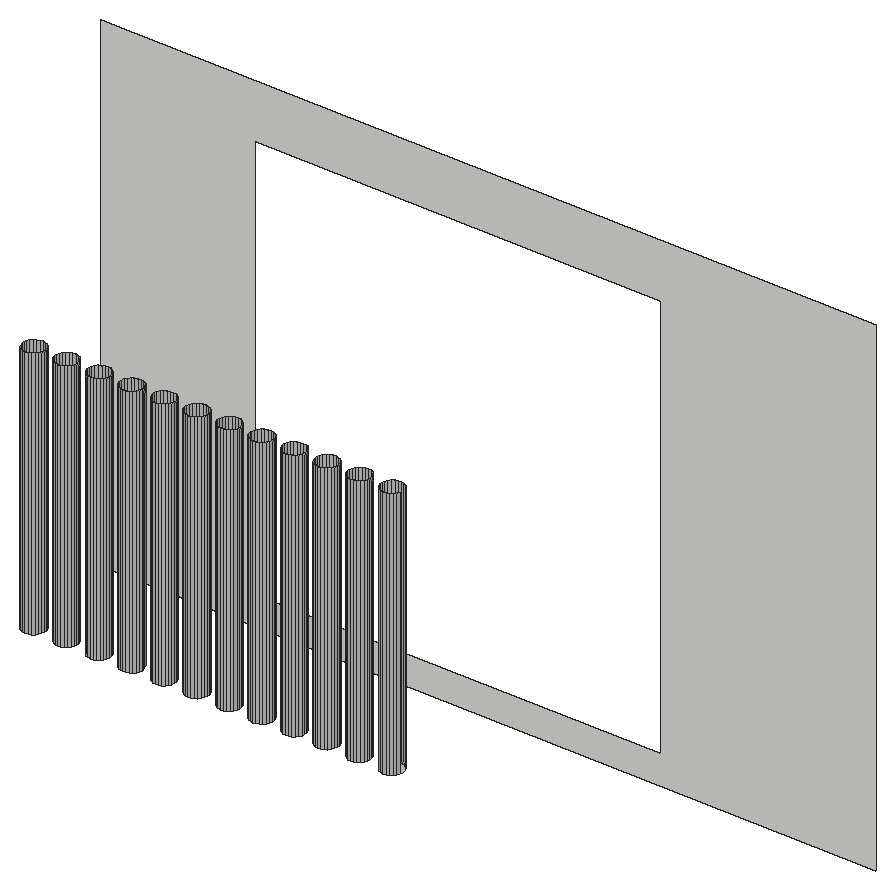
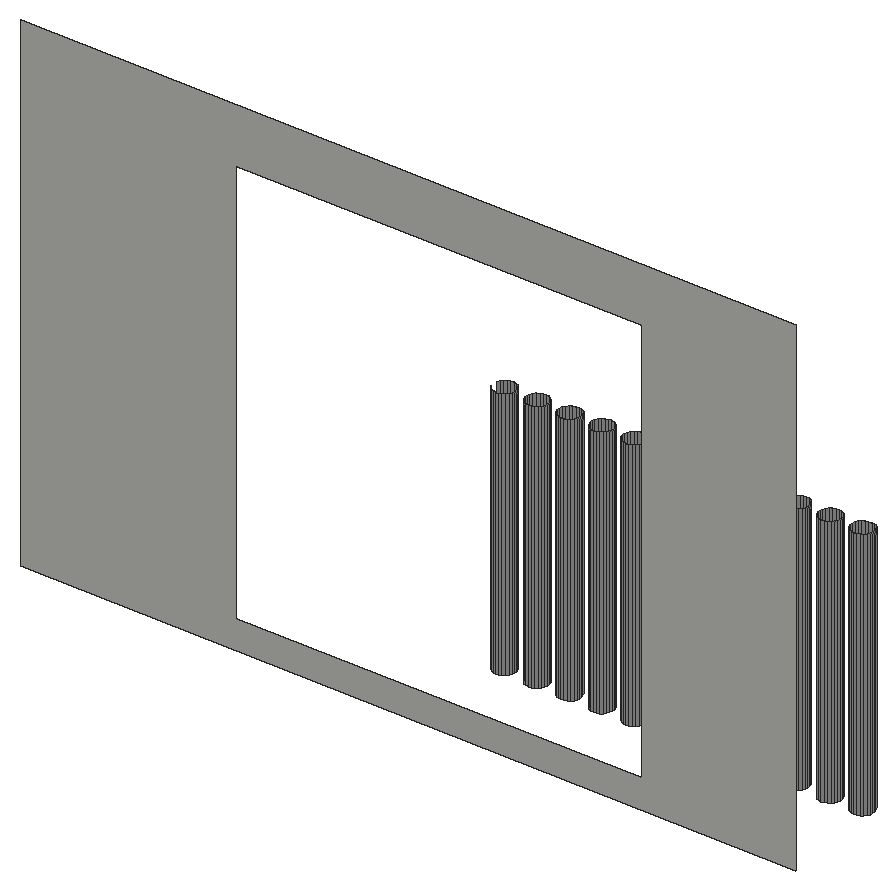
# SketchUp Ruby script. Lengths in millimetres.
U = 1.mm
M = Sketchup.active_model
def pt(a) = Geom::Point3d.new(a.map { |v| v * U })
def face(e, loops, mat)
  f = e.add_face(loops[0].map { |a| pt(a) })
  loops[1..].each { |l| e.add_face(l.map { |a| pt(a) }).erase! }
  f.material = f.back_material = mat if mat
  f
end
# faces: each face lists its corners as indices into pts; further lists are holes
def faces(e, pts, list, mat = nil) = list.each { |f| face(e, (f[0].is_a?(Array) ? f : [f]).map { |l| l.map { |i| pts[i] } }, mat) }
# xy, xz, yz: faces in a plane at the given z, y or x. An outline is a flat list of corners, or four numbers for a rectangle; further outlines are holes
def ring(l) = l.size == 4 ? [[l[0], l[1]], [l[2], l[1]], [l[2], l[3]], [l[0], l[3]]] : l.each_slice(2).to_a
def flat(e, list, mat, &to3) = list.each { |f| face(e, (f[0].is_a?(Array) ? f : [f]).map { |l| ring(l).map { |u, v| to3.(u, v) } }, mat) }
def xy(e, z, list, mat = nil) = flat(e, list, mat) { |x, y| [x, y, z] }
def xz(e, y, list, mat = nil) = flat(e, list, mat) { |x, z| [x, y, z] }
def yz(e, x, list, mat = nil) = flat(e, list, mat) { |y, z| [x, y, z] }
def lines(e, pts, list) = list.each { |a, b| e.add_line(pt(pts[a]), pt(pts[b])) }
# prism: a flat outline (further loops are holes) pulled along v
def prism(e, loops, v, mat = nil)
  f = face(e, loops, mat); d = Geom::Vector3d.new(v.map { |x| x * U })
  f.pushpull(f.normal.samedirection?(d) ? d.length : -d.length)
end
def box(e, o, s, mat = nil) = prism(e, [[o, [o[0] + s[0], o[1], o[2]], [o[0] + s[0], o[1] + s[1], o[2]], [o[0], o[1] + s[1], o[2]]]], [0, 0, s[2]], mat)
def at(x, y, z, deg = 0) = Geom::Transformation.translation(pt([x, y, z])) * Geom::Transformation.rotation(ORIGIN, Z_AXIS, deg.degrees)
def axes(o, x, y, z) = Geom::Transformation.new([*x, 0, *y, 0, *z, 0, *pt(o).to_a, 1])
def part(name) = M.definitions.add(name)
# library, detail: a bought-in or finely detailed component or shape, given as its bounding box
def library(name, o, s) = part(name).tap { |d| box(d.entities, o, s) }
def detail(e, o, s) = box(e.add_group.entities, o, s)
def put(e, d, t, mat = nil) = e.add_instance(d, t).tap { |i| i.material = mat if mat }
def group(e, t, mat = nil) = e.add_group.tap { |g| g.transformation = t; g.material = mat if mat }.entities
root = M.entities
M.materials.add("[Metal Corrugated Shiny]").color = [193, 193, 193]
xy(root,3899.4,[[7323,932.9,7306.2,935.4,7290.6,942.1,7277.2,952.6,7267.1,966.2,7260.8,982,7258.8,998.9,7261.3,1015.7,7268,1031.3,7278.5,1044.7,7292.1,1054.8,7307.9,1061.1,7324.8,1063.1,7341.6,1060.6,7357.2,1053.9,7370.6,1043.4,7380.7,1029.8,7387,1014,7389,997.1,7386.5,980.3,7379.8,964.7,7369.3,951.3,7355.7,941.2,7339.9,934.9],[7519.8,932.9,7503,935.4,7487.4,942.1,7474.1,952.6,7463.9,966.2,7457.6,982,7455.7,998.9,7458.1,1015.7,7464.8,1031.3,7475.4,1044.7,7489,1054.8,7504.8,1061.1,7521.6,1063.1,7538.5,1060.6,7554.1,1053.9,7567.4,1043.4,7577.6,1029.8,7583.8,1014,7585.8,997.1,7583.4,980.3,7576.7,964.7,7566.1,951.3,7552.5,941.2,7536.7,934.9],[7716.7,932.9,7699.9,935.4,7684.3,942.1,7670.9,952.6,7660.8,966.2,7654.5,982,7652.5,998.9,7655,1015.7,7661.7,1031.3,7672.2,1044.7,7685.8,1054.8,7701.6,1061.1,7718.5,1063.1,7735.3,1060.6,7750.9,1053.9,7764.3,1043.4,7774.4,1029.8,7780.7,1014,7782.7,997.1,7780.2,980.3,7773.5,964.7,7763,951.3,7749.4,941.2,7733.6,934.9],[7913.5,932.9,7896.7,935.4,7881.1,942.1,7867.8,952.6,7857.6,966.2,7851.3,982,7849.4,998.9,7851.8,1015.7,7858.5,1031.3,7869.1,1044.7,7882.7,1054.8,7898.5,1061.1,7915.3,1063.1,7932.2,1060.6,7947.8,1053.9,7961.1,1043.4,7971.3,1029.8,7977.5,1014,7979.5,997.1,7977.1,980.3,7970.4,964.7,7959.8,951.3,7946.2,941.2,7930.4,934.9],[8110.4,932.9,8093.6,935.4,8078,942.1,8064.6,952.6,8054.5,966.2,8048.2,982,8046.2,998.9,8048.7,1015.7,8055.4,1031.3,8065.9,1044.7,8079.5,1054.8,8095.3,1061.1,8112.2,1063.1,8129,1060.6,8144.6,1053.9,8158,1043.4,8168.1,1029.8,8174.4,1014,8176.4,997.1,8173.9,980.3,8167.2,964.7,8156.7,951.3,8143.1,941.2,8127.3,934.9],
  [8307.2,932.9,8290.4,935.4,8274.8,942.1,8261.5,952.6,8251.3,966.2,8245,982,8243.1,998.9,8245.5,1015.7,8252.2,1031.3,8262.8,1044.7,8276.4,1054.8,8292.2,1061.1,8309,1063.1,8325.9,1060.6,8341.5,1053.9,8354.8,1043.4,8365,1029.8,8371.2,1014,8373.2,997.1,8370.8,980.3,8364.1,964.7,8353.5,951.3,8339.9,941.2,8324.1,934.9],[8504.1,932.9,8487.3,935.4,8471.7,942.1,8458.3,952.6,8448.2,966.2,8441.9,982,8439.9,998.9,8442.4,1015.7,8449.1,1031.3,8459.6,1044.7,8473.2,1054.8,8489,1061.1,8505.9,1063.1,8522.7,1060.6,8538.3,1053.9,8551.7,1043.4,8561.8,1029.8,8568.1,1014,8570.1,997.1,8567.6,980.3,8560.9,964.7,8550.4,951.3,8536.8,941.2,8521,934.9],[8700.9,932.9,8684.1,935.4,8668.5,942.1,8655.2,952.6,8645,966.2,8638.7,982,8636.8,998.9,8639.2,1015.7,8645.9,1031.3,8656.5,1044.7,8670.1,1054.8,8685.9,1061.1,8702.7,1063.1,8719.6,1060.6,8735.2,1053.9,8748.5,1043.4,8758.7,1029.8,8764.9,1014,8766.9,997.1,8764.5,980.3,8757.8,964.7,8747.2,951.3,8733.6,941.2,8717.8,934.9],[8897.8,932.9,8881,935.4,8865.4,942.1,8852,952.6,8841.9,966.2,8835.6,982,8833.6,998.9,8836.1,1015.7,8842.8,1031.3,8853.3,1044.7,8866.9,1054.8,8882.7,1061.1,8899.6,1063.1,8916.4,1060.6,8932,1053.9,8945.4,1043.4,8955.5,1029.8,8961.8,1014,8963.8,997.1,8961.3,980.3,8954.6,964.7,8944.1,951.3,8930.5,941.2,8914.7,934.9],[9094.6,932.9,9077.8,935.4,9062.2,942.1,9048.9,952.6,9038.7,966.2,9032.4,982,9030.5,998.9,9032.9,1015.7,9039.6,1031.3,9050.2,1044.7,9063.8,1054.8,9079.6,1061.1,9096.4,1063.1,9113.3,1060.6,9128.9,1053.9,9142.2,1043.4,9152.4,1029.8,9158.6,1014,9160.6,997.1,9158.2,980.3,9151.5,964.7,9140.9,951.3,9127.3,941.2,9111.5,934.9],
  [9291.5,932.9,9274.7,935.4,9259.1,942.1,9245.7,952.6,9235.6,966.2,9229.3,982,9227.3,998.9,9229.8,1015.7,9236.5,1031.3,9247,1044.7,9260.6,1054.8,9276.4,1061.1,9293.3,1063.1,9310.1,1060.6,9325.7,1053.9,9339.1,1043.4,9349.2,1029.8,9355.5,1014,9357.5,997.1,9355,980.3,9348.3,964.7,9337.8,951.3,9324.2,941.2,9308.4,934.9],[9488.3,932.9,9471.5,935.4,9455.9,942.1,9442.6,952.6,9432.4,966.2,9426.1,982,9424.2,998.9,9426.6,1015.7,9433.3,1031.3,9443.9,1044.7,9457.5,1054.8,9473.3,1061.1,9490.1,1063.1,9507,1060.6,9522.6,1053.9,9535.9,1043.4,9546.1,1029.8,9552.3,1014,9554.3,997.1,9551.9,980.3,9545.2,964.7,9534.6,951.3,9521,941.2,9505.2,934.9]],"[Metal Corrugated Shiny]")
xz(root,1657.4,[[[7199.4,3899.4,11890.5,6858],[8130.9,4073.5,10586.8,6529.3]]])
p = [[7306.2,935.4,3899.4],[7323,932.9,3899.4],[7323,932.9,5423.4],[7306.2,935.4,5423.4],[7339.9,934.9,3899.4],[7339.9,934.9,5423.4],
  [7503,935.4,3899.4],[7519.8,932.9,3899.4],[7519.8,932.9,5423.4],[7503,935.4,5423.4],[7536.7,934.9,3899.4],[7536.7,934.9,5423.4],
  [7699.9,935.4,3899.4],[7716.7,932.9,3899.4],[7716.7,932.9,5423.4],[7699.9,935.4,5423.4],[7733.6,934.9,3899.4],[7733.6,934.9,5423.4],
  [7896.7,935.4,3899.4],[7913.5,932.9,3899.4],[7913.5,932.9,5423.4],[7896.7,935.4,5423.4],[7930.4,934.9,3899.4],[7930.4,934.9,5423.4],
  [8093.6,935.4,3899.4],[8110.4,932.9,3899.4],[8110.4,932.9,5423.4],[8093.6,935.4,5423.4],[8127.3,934.9,3899.4],[8127.3,934.9,5423.4],
  [8290.4,935.4,3899.4],[8307.2,932.9,3899.4],[8307.2,932.9,5423.4],[8290.4,935.4,5423.4],[8324.1,934.9,3899.4],[8324.1,934.9,5423.4],
  [8487.3,935.4,3899.4],[8504.1,932.9,3899.4],[8504.1,932.9,5423.4],[8487.3,935.4,5423.4],[8521,934.9,3899.4],[8521,934.9,5423.4],
  [8684.1,935.4,3899.4],[8700.9,932.9,3899.4],[8700.9,932.9,5423.4],[8684.1,935.4,5423.4],[8717.8,934.9,3899.4],[8717.8,934.9,5423.4],
  [8881,935.4,3899.4],[8897.8,932.9,3899.4],[8897.8,932.9,5423.4],[8881,935.4,5423.4],[8914.7,934.9,3899.4],[8914.7,934.9,5423.4],
  [9077.8,935.4,3899.4],[9094.6,932.9,3899.4],[9094.6,932.9,5423.4],[9077.8,935.4,5423.4],[9111.5,934.9,3899.4],[9111.5,934.9,5423.4],
  [9274.7,935.4,3899.4],[9291.5,932.9,3899.4],[9291.5,932.9,5423.4],[9274.7,935.4,5423.4],[9308.4,934.9,3899.4],[9308.4,934.9,5423.4],
  [9471.5,935.4,3899.4],[9488.3,932.9,3899.4],[9488.3,932.9,5423.4],[9471.5,935.4,5423.4],[9505.2,934.9,3899.4],[9505.2,934.9,5423.4],
  [7355.7,941.2,3899.4],[7355.7,941.2,5423.4],[7552.5,941.2,3899.4],[7552.5,941.2,5423.4],[7749.4,941.2,3899.4],[7749.4,941.2,5423.4],
  [7946.2,941.2,3899.4],[7946.2,941.2,5423.4],[8143.1,941.2,3899.4],[8143.1,941.2,5423.4],[8339.9,941.2,3899.4],[8339.9,941.2,5423.4],
  [8536.8,941.2,3899.4],[8536.8,941.2,5423.4],[8733.6,941.2,3899.4],[8733.6,941.2,5423.4],[8930.5,941.2,3899.4],[8930.5,941.2,5423.4],
  [9127.3,941.2,3899.4],[9127.3,941.2,5423.4],[9324.2,941.2,3899.4],[9324.2,941.2,5423.4],[9521,941.2,3899.4],[9521,941.2,5423.4],
  [7290.6,942.1,3899.4],[7290.6,942.1,5423.4],[7487.4,942.1,3899.4],[7487.4,942.1,5423.4],[7684.3,942.1,3899.4],[7684.3,942.1,5423.4],
  [7881.1,942.1,3899.4],[7881.1,942.1,5423.4],[8078,942.1,3899.4],[8078,942.1,5423.4],[8274.8,942.1,3899.4],[8274.8,942.1,5423.4],
  [8471.7,942.1,3899.4],[8471.7,942.1,5423.4],[8668.5,942.1,3899.4],[8668.5,942.1,5423.4],[8865.4,942.1,3899.4],[8865.4,942.1,5423.4],
  [9062.2,942.1,3899.4],[9062.2,942.1,5423.4],[9259.1,942.1,3899.4],[9259.1,942.1,5423.4],[9455.9,942.1,3899.4],[9455.9,942.1,5423.4],
  [7369.3,951.3,3899.4],[7369.3,951.3,5423.4],[7566.1,951.3,3899.4],[7566.1,951.3,5423.4],[7763,951.3,3899.4],[7763,951.3,5423.4],
  [7959.8,951.3,3899.4],[7959.8,951.3,5423.4],[8156.7,951.3,3899.4],[8156.7,951.3,5423.4],[8353.5,951.3,3899.4],[8353.5,951.3,5423.4],
  [8550.4,951.3,3899.4],[8550.4,951.3,5423.4],[8747.2,951.3,3899.4],[8747.2,951.3,5423.4],[8944.1,951.3,3899.4],[8944.1,951.3,5423.4],
  [9140.9,951.3,3899.4],[9140.9,951.3,5423.4],[9337.8,951.3,3899.4],[9337.8,951.3,5423.4],[9534.6,951.3,3899.4],[9534.6,951.3,5423.4],
  [7277.2,952.6,3899.4],[7277.2,952.6,5423.4],[7474.1,952.6,3899.4],[7474.1,952.6,5423.4],[7670.9,952.6,3899.4],[7670.9,952.6,5423.4],
  [7867.8,952.6,3899.4],[7867.8,952.6,5423.4],[8064.6,952.6,3899.4],[8064.6,952.6,5423.4],[8261.5,952.6,3899.4],[8261.5,952.6,5423.4],
  [8458.3,952.6,3899.4],[8458.3,952.6,5423.4],[8655.2,952.6,3899.4],[8655.2,952.6,5423.4],[8852,952.6,3899.4],[8852,952.6,5423.4],
  [9048.9,952.6,3899.4],[9048.9,952.6,5423.4],[9245.7,952.6,3899.4],[9245.7,952.6,5423.4],[9442.6,952.6,3899.4],[9442.6,952.6,5423.4],
  [7379.8,964.7,3899.4],[7379.8,964.7,5423.4],[7576.7,964.7,3899.4],[7576.7,964.7,5423.4],[7773.5,964.7,3899.4],[7773.5,964.7,5423.4],
  [7970.4,964.7,3899.4],[7970.4,964.7,5423.4],[8167.2,964.7,3899.4],[8167.2,964.7,5423.4],[8364.1,964.7,3899.4],[8364.1,964.7,5423.4],
  [8560.9,964.7,3899.4],[8560.9,964.7,5423.4],[8757.8,964.7,3899.4],[8757.8,964.7,5423.4],[8954.6,964.7,3899.4],[8954.6,964.7,5423.4],
  [9151.5,964.7,3899.4],[9151.5,964.7,5423.4],[9348.3,964.7,3899.4],[9348.3,964.7,5423.4],[9545.2,964.7,3899.4],[9545.2,964.7,5423.4],
  [7267.1,966.2,3899.4],[7267.1,966.2,5423.4],[7463.9,966.2,3899.4],[7463.9,966.2,5423.4],[7660.8,966.2,3899.4],[7660.8,966.2,5423.4],
  [7857.6,966.2,3899.4],[7857.6,966.2,5423.4],[8054.5,966.2,3899.4],[8054.5,966.2,5423.4],[8251.3,966.2,3899.4],[8251.3,966.2,5423.4],
  [8448.2,966.2,3899.4],[8448.2,966.2,5423.4],[8645,966.2,3899.4],[8645,966.2,5423.4],[8841.9,966.2,3899.4],[8841.9,966.2,5423.4],
  [9038.7,966.2,3899.4],[9038.7,966.2,5423.4],[9235.6,966.2,3899.4],[9235.6,966.2,5423.4],[9432.4,966.2,3899.4],[9432.4,966.2,5423.4],
  [7386.5,980.3,3899.4],[7386.5,980.3,5423.4],[7583.4,980.3,3899.4],[7583.4,980.3,5423.4],[7780.2,980.3,3899.4],[7780.2,980.3,5423.4],
  [7977.1,980.3,3899.4],[7977.1,980.3,5423.4],[8173.9,980.3,3899.4],[8173.9,980.3,5423.4],[8370.8,980.3,3899.4],[8370.8,980.3,5423.4],
  [8567.6,980.3,3899.4],[8567.6,980.3,5423.4],[8764.5,980.3,3899.4],[8764.5,980.3,5423.4],[8961.3,980.3,3899.4],[8961.3,980.3,5423.4],
  [9158.2,980.3,3899.4],[9158.2,980.3,5423.4],[9355,980.3,3899.4],[9355,980.3,5423.4],[9551.9,980.3,3899.4],[9551.9,980.3,5423.4],
  [7260.8,982,3899.4],[7260.8,982,5423.4],[7457.6,982,3899.4],[7457.6,982,5423.4],[7654.5,982,3899.4],[7654.5,982,5423.4],
  [7851.3,982,3899.4],[7851.3,982,5423.4],[8048.2,982,3899.4],[8048.2,982,5423.4],[8245,982,3899.4],[8245,982,5423.4],
  [8441.9,982,3899.4],[8441.9,982,5423.4],[8638.7,982,3899.4],[8638.7,982,5423.4],[8835.6,982,3899.4],[8835.6,982,5423.4],
  [9032.4,982,3899.4],[9032.4,982,5423.4],[9229.3,982,3899.4],[9229.3,982,5423.4],[9426.1,982,3899.4],[9426.1,982,5423.4],
  [7389,997.1,3899.4],[7389,997.1,5423.4],[7585.8,997.1,3899.4],[7585.8,997.1,5423.4],[7782.7,997.1,3899.4],[7782.7,997.1,5423.4],
  [7979.5,997.1,3899.4],[7979.5,997.1,5423.4],[8176.4,997.1,3899.4],[8176.4,997.1,5423.4],[8373.2,997.1,3899.4],[8373.2,997.1,5423.4],
  [8570.1,997.1,3899.4],[8570.1,997.1,5423.4],[8766.9,997.1,3899.4],[8766.9,997.1,5423.4],[8963.8,997.1,3899.4],[8963.8,997.1,5423.4],
  [9160.6,997.1,3899.4],[9160.6,997.1,5423.4],[9357.5,997.1,3899.4],[9357.5,997.1,5423.4],[7258.8,998.9,3899.4],[7258.8,998.9,5423.4],
  [7455.7,998.9,3899.4],[7455.7,998.9,5423.4],[7652.5,998.9,3899.4],[7652.5,998.9,5423.4],[7849.4,998.9,3899.4],[7849.4,998.9,5423.4],
  [8046.2,998.9,3899.4],[8046.2,998.9,5423.4],[8243.1,998.9,3899.4],[8243.1,998.9,5423.4],[8439.9,998.9,3899.4],[8439.9,998.9,5423.4],
  [8636.8,998.9,3899.4],[8636.8,998.9,5423.4],[8833.6,998.9,3899.4],[8833.6,998.9,5423.4],[9030.5,998.9,3899.4],[9030.5,998.9,5423.4],
  [9227.3,998.9,3899.4],[9227.3,998.9,5423.4],[9424.2,998.9,3899.4],[9424.2,998.9,5423.4],[7387,1014,3899.4],[7387,1014,5423.4],
  [7583.8,1014,3899.4],[7583.8,1014,5423.4],[7780.7,1014,3899.4],[7780.7,1014,5423.4],[7977.5,1014,3899.4],[7977.5,1014,5423.4],
  [8174.4,1014,3899.4],[8174.4,1014,5423.4],[8371.2,1014,3899.4],[8371.2,1014,5423.4],[8568.1,1014,3899.4],[8568.1,1014,5423.4],
  [8764.9,1014,3899.4],[8764.9,1014,5423.4],[8961.8,1014,3899.4],[8961.8,1014,5423.4],[9158.6,1014,3899.4],[9158.6,1014,5423.4],
  [9355.5,1014,3899.4],[9355.5,1014,5423.4],[7261.3,1015.7,3899.4],[7261.3,1015.7,5423.4],[7458.1,1015.7,3899.4],[7458.1,1015.7,5423.4],
  [7655,1015.7,3899.4],[7655,1015.7,5423.4],[7851.8,1015.7,3899.4],[7851.8,1015.7,5423.4],[8048.7,1015.7,3899.4],[8048.7,1015.7,5423.4],
  [8245.5,1015.7,3899.4],[8245.5,1015.7,5423.4],[8442.4,1015.7,3899.4],[8442.4,1015.7,5423.4],[8639.2,1015.7,3899.4],[8639.2,1015.7,5423.4],
  [8836.1,1015.7,3899.4],[8836.1,1015.7,5423.4],[9032.9,1015.7,3899.4],[9032.9,1015.7,5423.4],[9229.8,1015.7,3899.4],[9229.8,1015.7,5423.4],
  [9426.6,1015.7,3899.4],[9426.6,1015.7,5423.4],[7380.7,1029.8,3899.4],[7380.7,1029.8,5423.4],[7577.6,1029.8,3899.4],[7577.6,1029.8,5423.4],
  [7774.4,1029.8,3899.4],[7774.4,1029.8,5423.4],[7971.3,1029.8,3899.4],[7971.3,1029.8,5423.4],[8168.1,1029.8,3899.4],[8168.1,1029.8,5423.4],
  [8365,1029.8,3899.4],[8365,1029.8,5423.4],[8561.8,1029.8,3899.4],[8561.8,1029.8,5423.4],[8758.7,1029.8,3899.4],[8758.7,1029.8,5423.4],
  [8955.5,1029.8,3899.4],[8955.5,1029.8,5423.4],[9152.4,1029.8,3899.4],[9152.4,1029.8,5423.4],[9349.2,1029.8,3899.4],[9349.2,1029.8,5423.4],
  [7268,1031.3,3899.4],[7268,1031.3,5423.4],[7464.8,1031.3,3899.4],[7464.8,1031.3,5423.4],[7661.7,1031.3,3899.4],[7661.7,1031.3,5423.4],
  [7858.5,1031.3,3899.4],[7858.5,1031.3,5423.4],[8055.4,1031.3,3899.4],[8055.4,1031.3,5423.4],[8252.2,1031.3,3899.4],[8252.2,1031.3,5423.4],
  [8449.1,1031.3,3899.4],[8449.1,1031.3,5423.4],[8645.9,1031.3,3899.4],[8645.9,1031.3,5423.4],[8842.8,1031.3,3899.4],[8842.8,1031.3,5423.4],
  [9039.6,1031.3,3899.4],[9039.6,1031.3,5423.4],[9236.5,1031.3,3899.4],[9236.5,1031.3,5423.4],[9433.3,1031.3,3899.4],[9433.3,1031.3,5423.4],
  [7370.6,1043.4,3899.4],[7370.6,1043.4,5423.4],[7567.4,1043.4,3899.4],[7567.4,1043.4,5423.4],[7764.3,1043.4,3899.4],[7764.3,1043.4,5423.4],
  [7961.1,1043.4,3899.4],[7961.1,1043.4,5423.4],[8158,1043.4,3899.4],[8158,1043.4,5423.4],[8354.8,1043.4,3899.4],[8354.8,1043.4,5423.4],
  [8551.7,1043.4,3899.4],[8551.7,1043.4,5423.4],[8748.5,1043.4,3899.4],[8748.5,1043.4,5423.4],[8945.4,1043.4,3899.4],[8945.4,1043.4,5423.4],
  [9142.2,1043.4,3899.4],[9142.2,1043.4,5423.4],[9339.1,1043.4,3899.4],[9339.1,1043.4,5423.4],[9546.1,1029.8,3899.4],[9535.9,1043.4,3899.4],
  [9535.9,1043.4,5423.4],[9546.1,1029.8,5423.4],[7278.5,1044.7,3899.4],[7278.5,1044.7,5423.4],[7475.4,1044.7,3899.4],[7475.4,1044.7,5423.4],
  [7672.2,1044.7,3899.4],[7672.2,1044.7,5423.4],[7869.1,1044.7,3899.4],[7869.1,1044.7,5423.4],[8065.9,1044.7,3899.4],[8065.9,1044.7,5423.4],
  [8262.8,1044.7,3899.4],[8262.8,1044.7,5423.4],[8459.6,1044.7,3899.4],[8459.6,1044.7,5423.4],[8656.5,1044.7,3899.4],[8656.5,1044.7,5423.4],
  [8853.3,1044.7,3899.4],[8853.3,1044.7,5423.4],[9050.2,1044.7,3899.4],[9050.2,1044.7,5423.4],[9247,1044.7,3899.4],[9247,1044.7,5423.4],
  [9443.9,1044.7,3899.4],[9443.9,1044.7,5423.4],[7357.2,1053.9,3899.4],[7357.2,1053.9,5423.4],[7554.1,1053.9,3899.4],[7554.1,1053.9,5423.4],
  [7750.9,1053.9,3899.4],[7750.9,1053.9,5423.4],[7947.8,1053.9,3899.4],[7947.8,1053.9,5423.4],[8144.6,1053.9,3899.4],[8144.6,1053.9,5423.4],
  [8341.5,1053.9,3899.4],[8341.5,1053.9,5423.4],[8538.3,1053.9,3899.4],[8538.3,1053.9,5423.4],[8735.2,1053.9,3899.4],[8735.2,1053.9,5423.4],
  [8932,1053.9,3899.4],[8932,1053.9,5423.4],[9128.9,1053.9,3899.4],[9128.9,1053.9,5423.4],[9325.7,1053.9,3899.4],[9325.7,1053.9,5423.4],
  [9522.6,1053.9,3899.4],[9522.6,1053.9,5423.4],[7292.1,1054.8,3899.4],[7292.1,1054.8,5423.4],[7489,1054.8,3899.4],[7489,1054.8,5423.4],
  [7685.8,1054.8,3899.4],[7685.8,1054.8,5423.4],[7882.7,1054.8,3899.4],[7882.7,1054.8,5423.4],[8079.5,1054.8,3899.4],[8079.5,1054.8,5423.4],
  [8276.4,1054.8,3899.4],[8276.4,1054.8,5423.4],[8473.2,1054.8,3899.4],[8473.2,1054.8,5423.4],[8670.1,1054.8,3899.4],[8670.1,1054.8,5423.4],
  [8866.9,1054.8,3899.4],[8866.9,1054.8,5423.4],[9063.8,1054.8,3899.4],[9063.8,1054.8,5423.4],[9260.6,1054.8,3899.4],[9260.6,1054.8,5423.4],
  [9457.5,1054.8,3899.4],[9457.5,1054.8,5423.4],[7341.6,1060.6,3899.4],[7341.6,1060.6,5423.4],[7538.5,1060.6,3899.4],[7538.5,1060.6,5423.4],
  [7735.3,1060.6,3899.4],[7735.3,1060.6,5423.4],[7932.2,1060.6,3899.4],[7932.2,1060.6,5423.4],[8129,1060.6,3899.4],[8129,1060.6,5423.4],
  [8325.9,1060.6,3899.4],[8325.9,1060.6,5423.4],[8522.7,1060.6,3899.4],[8522.7,1060.6,5423.4],[8719.6,1060.6,3899.4],[8719.6,1060.6,5423.4],
  [8916.4,1060.6,3899.4],[8916.4,1060.6,5423.4],[9113.3,1060.6,3899.4],[9113.3,1060.6,5423.4],[9310.1,1060.6,3899.4],[9310.1,1060.6,5423.4],
  [9507,1060.6,3899.4],[9507,1060.6,5423.4],[7307.9,1061.1,3899.4],[7307.9,1061.1,5423.4],[7504.8,1061.1,3899.4],[7504.8,1061.1,5423.4],
  [7701.6,1061.1,3899.4],[7701.6,1061.1,5423.4],[7898.5,1061.1,3899.4],[7898.5,1061.1,5423.4],[8095.3,1061.1,3899.4],[8095.3,1061.1,5423.4],
  [8292.2,1061.1,3899.4],[8292.2,1061.1,5423.4],[8489,1061.1,3899.4],[8489,1061.1,5423.4],[8685.9,1061.1,3899.4],[8685.9,1061.1,5423.4],
  [8882.7,1061.1,3899.4],[8882.7,1061.1,5423.4],[9079.6,1061.1,3899.4],[9079.6,1061.1,5423.4],[9276.4,1061.1,3899.4],[9276.4,1061.1,5423.4],
  [9473.3,1061.1,3899.4],[9473.3,1061.1,5423.4],[7324.8,1063.1,3899.4],[7324.8,1063.1,5423.4],[7521.6,1063.1,3899.4],[7521.6,1063.1,5423.4],
  [7718.5,1063.1,3899.4],[7718.5,1063.1,5423.4],[7915.3,1063.1,3899.4],[7915.3,1063.1,5423.4],[8112.2,1063.1,3899.4],[8112.2,1063.1,5423.4],
  [8309,1063.1,3899.4],[8309,1063.1,5423.4],[8505.9,1063.1,3899.4],[8505.9,1063.1,5423.4],[8702.7,1063.1,3899.4],[8702.7,1063.1,5423.4],
  [8899.6,1063.1,3899.4],[8899.6,1063.1,5423.4],[9096.4,1063.1,3899.4],[9096.4,1063.1,5423.4],[9293.3,1063.1,3899.4],[9293.3,1063.1,5423.4],
  [9490.1,1063.1,3899.4],[9490.1,1063.1,5423.4]]
faces(root,p,[[0,1,2,3],[1,4,5,2],[6,7,8,9],[7,10,11,8],[12,13,14,15],[13,16,17,14],[18,19,20,21],[19,22,23,20],
  [24,25,26,27],[25,28,29,26],[30,31,32,33],[31,34,35,32],[36,37,38,39],[37,40,41,38],[42,43,44,45],[43,46,47,44],
  [48,49,50,51],[49,52,53,50],[54,55,56,57],[55,58,59,56],[60,61,62,63],[61,64,65,62],[66,67,68,69],[67,70,71,68],
  [4,72,73,5],[10,74,75,11],[16,76,77,17],[22,78,79,23],[28,80,81,29],[34,82,83,35],[40,84,85,41],[46,86,87,47],
  [52,88,89,53],[58,90,91,59],[64,92,93,65],[70,94,95,71],[96,0,3,97],[98,6,9,99],[100,12,15,101],[102,18,21,103],
  [104,24,27,105],[106,30,33,107],[108,36,39,109],[110,42,45,111],[112,48,51,113],[114,54,57,115],[116,60,63,117],[118,66,69,119],
  [72,120,121,73],[74,122,123,75],[76,124,125,77],[78,126,127,79],[80,128,129,81],[82,130,131,83],[84,132,133,85],[86,134,135,87],
  [88,136,137,89],[90,138,139,91],[92,140,141,93],[94,142,143,95],[144,96,97,145],[146,98,99,147],[148,100,101,149],[150,102,103,151],
  [152,104,105,153],[154,106,107,155],[156,108,109,157],[158,110,111,159],[160,112,113,161],[162,114,115,163],[164,116,117,165],[166,118,119,167],
  [120,168,169,121],[122,170,171,123],[124,172,173,125],[126,174,175,127],[128,176,177,129],[130,178,179,131],[132,180,181,133],[134,182,183,135],
  [136,184,185,137],[138,186,187,139],[140,188,189,141],[142,190,191,143],[192,144,145,193],[194,146,147,195],[196,148,149,197],[198,150,151,199],
  [200,152,153,201],[202,154,155,203],[204,156,157,205],[206,158,159,207],[208,160,161,209],[210,162,163,211],[212,164,165,213],[214,166,167,215],
  [168,216,217,169],[170,218,219,171],[172,220,221,173],[174,222,223,175],[176,224,225,177],[178,226,227,179],[180,228,229,181],[182,230,231,183],
  [184,232,233,185],[186,234,235,187],[188,236,237,189],[190,238,239,191],[240,192,193,241],[242,194,195,243],[244,196,197,245],[246,198,199,247],
  [248,200,201,249],[250,202,203,251],[252,204,205,253],[254,206,207,255],[256,208,209,257],[258,210,211,259],[260,212,213,261],[262,214,215,263],
  [216,264,265,217],[218,266,267,219],[220,268,269,221],[222,270,271,223],[224,272,273,225],[226,274,275,227],[228,276,277,229],[230,278,279,231],
  [232,280,281,233],[234,282,283,235],[236,284,285,237],[286,240,241,287],[288,242,243,289],[290,244,245,291],[292,246,247,293],[294,248,249,295],
  [296,250,251,297],[298,252,253,299],[300,254,255,301],[302,256,257,303],[304,258,259,305],[306,260,261,307],[308,262,263,309],[264,310,311,265],
  [266,312,313,267],[268,314,315,269],[270,316,317,271],[272,318,319,273],[274,320,321,275],[276,322,323,277],[278,324,325,279],[280,326,327,281],
  [282,328,329,283],[284,330,331,285],[332,286,287,333],[334,288,289,335],[336,290,291,337],[338,292,293,339],[340,294,295,341],[342,296,297,343],
  [344,298,299,345],[346,300,301,347],[348,302,303,349],[350,304,305,351],[352,306,307,353],[354,308,309,355],[310,356,357,311],[312,358,359,313],
  [314,360,361,315],[316,362,363,317],[318,364,365,319],[320,366,367,321],[322,368,369,323],[324,370,371,325],[326,372,373,327],[328,374,375,329],
  [330,376,377,331],[378,332,333,379],[380,334,335,381],[382,336,337,383],[384,338,339,385],[386,340,341,387],[388,342,343,389],[390,344,345,391],
  [392,346,347,393],[394,348,349,395],[396,350,351,397],[398,352,353,399],[400,354,355,401],[356,402,403,357],[358,404,405,359],[360,406,407,361],
  [362,408,409,363],[364,410,411,365],[366,412,413,367],[368,414,415,369],[370,416,417,371],[372,418,419,373],[374,420,421,375],[376,422,423,377],
  [424,425,426,427],[428,378,379,429],[430,380,381,431],[432,382,383,433],[434,384,385,435],[436,386,387,437],[438,388,389,439],[440,390,391,441],
  [442,392,393,443],[444,394,395,445],[446,396,397,447],[448,398,399,449],[450,400,401,451],[402,452,453,403],[404,454,455,405],[406,456,457,407],
  [408,458,459,409],[410,460,461,411],[412,462,463,413],[414,464,465,415],[416,466,467,417],[418,468,469,419],[420,470,471,421],[422,472,473,423],
  [425,474,475,426],[476,428,429,477],[478,430,431,479],[480,432,433,481],[482,434,435,483],[484,436,437,485],[486,438,439,487],[488,440,441,489],
  [490,442,443,491],[492,444,445,493],[494,446,447,495],[496,448,449,497],[498,450,451,499],[452,500,501,453],[454,502,503,455],[456,504,505,457],
  [458,506,507,459],[460,508,509,461],[462,510,511,463],[464,512,513,465],[466,514,515,467],[468,516,517,469],[470,518,519,471],[472,520,521,473],
  [474,522,523,475],[524,476,477,525],[526,478,479,527],[528,480,481,529],[530,482,483,531],[532,484,485,533],[534,486,487,535],[536,488,489,537],
  [538,490,491,539],[540,492,493,541],[542,494,495,543],[544,496,497,545],[546,498,499,547],[500,548,549,501],[502,550,551,503],[504,552,553,505],
  [506,554,555,507],[508,556,557,509],[510,558,559,511],[512,560,561,513],[514,562,563,515],[516,564,565,517],[518,566,567,519],[520,568,569,521],
  [522,570,571,523],[548,524,525,549],[550,526,527,551],[552,528,529,553],[554,530,531,555],[556,532,533,557],[558,534,535,559],[560,536,537,561],
  [562,538,539,563],[564,540,541,565],[566,542,543,567],[568,544,545,569],[570,546,547,571]],"[Metal Corrugated Shiny]")
